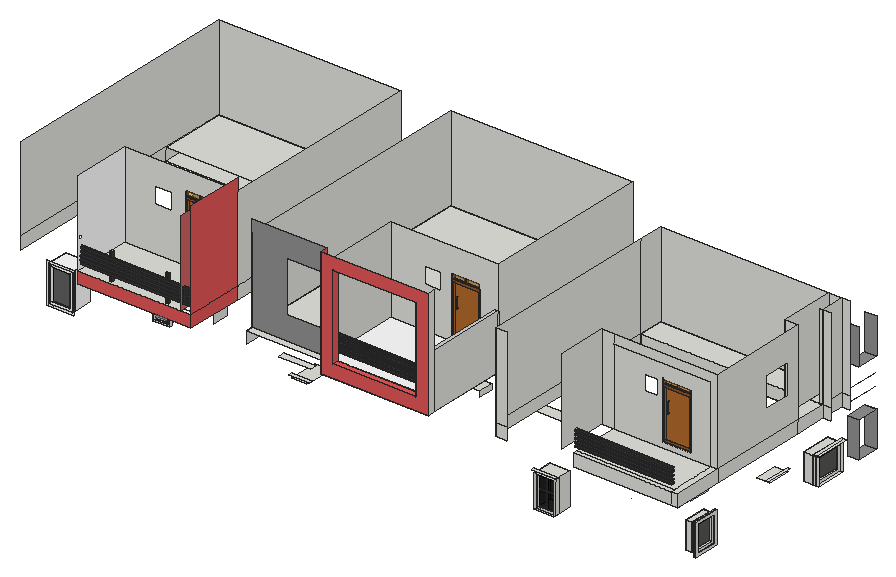
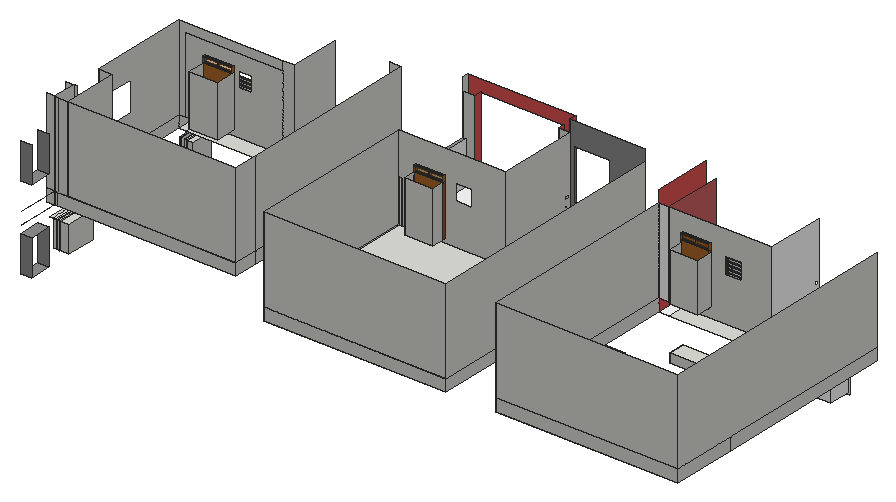
# SketchUp Ruby script. Lengths in inches.
U = 1.inch
M = Sketchup.active_model
def pt(a) = Geom::Point3d.new(a.map { |v| v * U })
def face(e, loops, mat)
  f = e.add_face(loops[0].map { |a| pt(a) })
  loops[1..].each { |l| e.add_face(l.map { |a| pt(a) }).erase! }
  f.material = f.back_material = mat if mat
  f
end
# faces: each face lists its corners as indices into pts; further lists are holes
def faces(e, pts, list, mat = nil) = list.each { |f| face(e, (f[0].is_a?(Array) ? f : [f]).map { |l| l.map { |i| pts[i] } }, mat) }
# xy, xz, yz: faces in a plane at the given z, y or x. An outline is a flat list of corners, or four numbers for a rectangle; further outlines are holes
def ring(l) = l.size == 4 ? [[l[0], l[1]], [l[2], l[1]], [l[2], l[3]], [l[0], l[3]]] : l.each_slice(2).to_a
def flat(e, list, mat, &to3) = list.each { |f| face(e, (f[0].is_a?(Array) ? f : [f]).map { |l| ring(l).map { |u, v| to3.(u, v) } }, mat) }
def xy(e, z, list, mat = nil) = flat(e, list, mat) { |x, y| [x, y, z] }
def xz(e, y, list, mat = nil) = flat(e, list, mat) { |x, z| [x, y, z] }
def yz(e, x, list, mat = nil) = flat(e, list, mat) { |y, z| [x, y, z] }
def lines(e, pts, list) = list.each { |a, b| e.add_line(pt(pts[a]), pt(pts[b])) }
# prism: a flat outline (further loops are holes) pulled along v
def prism(e, loops, v, mat = nil)
  f = face(e, loops, mat); d = Geom::Vector3d.new(v.map { |x| x * U })
  f.pushpull(f.normal.samedirection?(d) ? d.length : -d.length)
end
def box(e, o, s, mat = nil) = prism(e, [[o, [o[0] + s[0], o[1], o[2]], [o[0] + s[0], o[1] + s[1], o[2]], [o[0], o[1] + s[1], o[2]]]], [0, 0, s[2]], mat)
def at(x, y, z, deg = 0) = Geom::Transformation.translation(pt([x, y, z])) * Geom::Transformation.rotation(ORIGIN, Z_AXIS, deg.degrees)
def axes(o, x, y, z) = Geom::Transformation.new([*x, 0, *y, 0, *z, 0, *pt(o).to_a, 1])
def part(name) = M.definitions.add(name)
# library, detail: a bought-in or finely detailed component or shape, given as its bounding box
def library(name, o, s) = part(name).tap { |d| box(d.entities, o, s) }
def detail(e, o, s) = box(e.add_group.entities, o, s)
def put(e, d, t, mat = nil) = e.add_instance(d, t).tap { |i| i.material = mat if mat }
def group(e, t, mat = nil) = e.add_group.tap { |g| g.transformation = t; g.material = mat if mat }.entities
root = M.entities
M.materials.add("Generic").color = [145, 145, 145]
M.materials.add("Generic\#1").color = [206, 99, 99]
M.materials.add("Generic\#2").color = [229, 87, 87]
M.materials.add("[Color M00]").color = [255, 255, 255]
M.materials.add("[Color M07]").color = [58, 58, 58]
M.materials.add("[Color M08]").color = [45, 45, 45]
M.materials.add("[Translucent Glass Dark Green]").color = [168, 100, 12]
M.materials["[Translucent Glass Dark Green]"].alpha = 0.5
M.materials.add("[Translucent Glass Gray]").color = [0, 0, 0]
M.materials["[Translucent Glass Gray]"].alpha = 0.62
M.materials.add("[Translucent Glass Gray]1").color = [128, 128, 128]
M.materials["[Translucent Glass Gray]1"].alpha = 0.5
M.materials.add("[Wood Bamboo]").color = [177, 105, 43]
M.materials.add("[Wood Cherry Original]").color = [152, 86, 42]
c1 = part("Group\#1")
xy(c1.entities,0,[[0,0,39.9375,6]])
xy(c1.entities,3.79,[[3.79,0,36.15,3]])
xy(c1.entities,60.83,[[3.79,0,36.15,3]])
xy(c1.entities,64.62,[[0,0,39.9375,6]])
xz(c1.entities,0,[[[0,0,39.9375,64.62],[3.79,3.79,36.15,60.83]]])
xz(c1.entities,3,[[18.07,3.79,20.49,3.79,20.49,32.1,36.15,32.1,36.15,34.21,20.49,34.21,20.49,60.83,18.07,60.83,18.07,34.21,3.79,34.21,3.79,32.1,18.07,32.1]],"[Color M08]")
xz(c1.entities,3,[[3.79,3.79,18.07,32.1],[20.49,3.79,36.15,32.1],[3.79,34.21,18.07,60.83],[20.49,34.21,36.15,60.83]],"[Translucent Glass Gray]")
xz(c1.entities,6,[[0,0,39.9375,64.62]],"[Translucent Glass Gray]")
yz(c1.entities,0,[[0,0,6,64.62]])
yz(c1.entities,3.79,[[0,3.79,3,60.83]])
yz(c1.entities,36.15,[[0,3.79,3,60.83]])
yz(c1.entities,39.9375,[[0,0,6,64.62]])
c2 = part("Group\#8")
xy(c2.entities,0,[[0,0,6,59.4375]])
xy(c2.entities,4.64,[[3,4.64,6,54.8]])
xy(c2.entities,46.99,[[3,4.64,6,54.8]])
xy(c2.entities,51.625,[[0,0,6,59.4375]])
xz(c2.entities,0,[[0,0,6,51.625]])
xz(c2.entities,4.64,[[3,4.64,6,46.99]])
xz(c2.entities,54.8,[[3,4.64,6,46.99]])
xz(c2.entities,59.4375,[[0,0,6,51.625]])
yz(c2.entities,0,[[0,0,59.4375,51.625]])
yz(c2.entities,3,[[4.64,4.64,54.8,46.99]],"[Translucent Glass Gray]")
yz(c2.entities,6,[[[0,0,59.4375,51.625],[4.64,4.64,54.8,46.99]]])
c3 = part("Group\#11")
xy(c3.entities,0,[[0,0,27.8125,3]])
xy(c3.entities,27.8125,[[0,0,27.8125,3]])
xz(c3.entities,0,[[0,0,27.8125,27.8125]],"[Translucent Glass Gray]1")
xz(c3.entities,3,[[0,0,27.8125,27.8125]],"[Translucent Glass Gray]1")
yz(c3.entities,0,[[0,0,3,27.8125]])
yz(c3.entities,27.8125,[[0,0,3,27.8125]])
c4 = part("Group\#7")
xy(c4.entities,0,[[0,0,6,43.1875]])
xy(c4.entities,3.45,[[3,3.45,6,39.74]])
xy(c4.entities,49.61,[[3,3.45,6,39.74]])
xy(c4.entities,53.0625,[[0,0,6,43.1875]])
xz(c4.entities,0,[[0,0,6,53.0625]])
xz(c4.entities,3.45,[[3,3.45,6,49.61]])
xz(c4.entities,39.74,[[3,3.45,6,49.61]])
xz(c4.entities,43.1875,[[0,0,6,53.0625]])
yz(c4.entities,0,[[0,0,43.1875,53.0625]])
yz(c4.entities,3,[[3.45,3.45,39.74,49.61]],"[Translucent Glass Gray]")
yz(c4.entities,6,[[[0,0,43.1875,53.0625],[3.45,3.45,39.74,49.61]]])
c5 = part("Group\#5")
xy(c5.entities,0,[[0,0,46.6875,6]],"[Color M00]")
xy(c5.entities,4.48,[[4.48,0,42.2,3]],"[Color M00]")
xy(c5.entities,67.45,[[4.48,0,42.2,3]],"[Color M00]")
xy(c5.entities,71.9375,[[0,0,46.6875,6]],"[Color M00]")
xz(c5.entities,0,[[[0,0,46.6875,71.9375],[4.48,4.48,42.2,67.45]]],"[Color M00]")
xz(c5.entities,3,[[4.48,4.48,42.2,67.45]],"[Translucent Glass Gray]")
xz(c5.entities,6,[[0,0,46.6875,71.9375]],"[Color M00]")
yz(c5.entities,0,[[0,0,6,71.9375]],"[Color M00]")
yz(c5.entities,4.48,[[0,4.48,3,67.45]],"[Color M00]")
yz(c5.entities,42.2,[[0,4.48,3,67.45]],"[Color M00]")
yz(c5.entities,46.6875,[[0,0,6,71.9375]],"[Color M00]")
c6 = part("Group\#12")
xy(c6.entities,0,[[0,0,20.25,3]])
xy(c6.entities,24.8125,[[0,0,20.25,3]])
xz(c6.entities,0,[[0,0,20.25,24.8125]],"[Translucent Glass Gray]1")
xz(c6.entities,3,[[0,0,20.25,24.8125]],"[Translucent Glass Gray]1")
yz(c6.entities,0,[[0,0,3,24.8125]])
yz(c6.entities,20.25,[[0,0,3,24.8125]])
c7 = part("Group\#10")
xy(c7.entities,0,[[0,1.08,55.8125,6.01]],"[Wood Cherry Original]")
xy(c7.entities,3.96,[[3.96,1.08,51.86,3.01]],"[Wood Bamboo]")
xy(c7.entities,51.66,[[8.63,0,9.88,3.01]],"[Color M08]")
xy(c7.entities,52.54,[[8.63,0.6875,9.88,3.01]],"[Color M08]")
xy(c7.entities,71.82,[[8.63,0.6875,9.88,3.01]],"[Color M08]")
xy(c7.entities,72.69,[[8.63,0,9.88,3.01]],"[Color M08]")
xy(c7.entities,97.36,[[3.96,1.08,51.86,3.01]],"[Wood Bamboo]")
xy(c7.entities,101.3125,[[0,1.08,55.8125,6.01]],"[Wood Bamboo]")
xy(c7.entities,102.55,[[1.23,1.08,27.29,3.01],[27.29,1.08,28.52,1.95],[28.52,1.08,54.58,3.01]],"[Wood Bamboo]")
xy(c7.entities,112.31,[[1.23,1.08,1.23,3.01,27.29,3.01,27.29,1.95,28.52,1.95,28.52,3.01,54.58,3.01,54.58,1.08]],"[Wood Bamboo]")
xy(c7.entities,113.54,[[0,1.08,55.8125,6.01]],"[Wood Bamboo]")
xz(c7.entities,0,[[8.63,51.66,9.88,72.69]],"[Color M08]")
xz(c7.entities,0.6875,[[8.63,52.54,9.88,71.82]])
xz(c7.entities,1.08,[[0,101.3125,55.8125,102.55],[0,102.55,1.23,102.55,1.23,112.31,54.58,112.31,54.58,102.55,55.8125,102.55,55.8125,113.54,0,113.54]],"[Wood Bamboo]")
xz(c7.entities,1.08,[[[0,0,55.8125,101.3125],[3.96,3.96,51.86,97.36]]],"[Wood Cherry Original]")
xz(c7.entities,1.95,[[27.29,102.55,28.52,112.31]],"[Wood Bamboo]")
xz(c7.entities,3.01,[[8.63,71.82,9.88,72.69]])
xz(c7.entities,3.01,[[1.23,102.55,27.29,112.31],[28.52,102.55,54.58,112.31]],"[Translucent Glass Dark Green]")
xz(c7.entities,3.01,[[[3.96,3.96,51.86,97.36],[8.63,71.82,9.88,72.69],[8.63,51.66,9.88,52.54]]],"[Wood Bamboo]")
xz(c7.entities,6.01,[[0,0,55.8125,101.3125],[0,112.31,55.8125,113.54]],"[Wood Bamboo]")
yz(c7.entities,0,[[1.08,101.3125,6.01,113.54]],"[Wood Bamboo]")
yz(c7.entities,0,[[1.08,0,6.01,101.3125]],"[Wood Cherry Original]")
yz(c7.entities,1.23,[[1.08,102.55,3.01,112.31]],"[Wood Bamboo]")
yz(c7.entities,3.96,[[1.08,3.96,3.01,97.36]],"[Wood Bamboo]")
yz(c7.entities,8.63,[[0,51.66,0,72.69,3.01,72.69,3.01,71.82,0.6875,71.82,0.6875,52.54,3.01,52.54,3.01,51.66]],"[Color M08]")
yz(c7.entities,9.88,[[0,51.66,3.01,51.66,3.01,52.54,0.6875,52.54,0.6875,71.82,3.01,71.82,3.01,72.69,0,72.69]],"[Color M08]")
yz(c7.entities,27.29,[[1.95,102.55,3.01,112.31]],"[Wood Bamboo]")
yz(c7.entities,28.52,[[1.95,102.55,3.01,112.31]],"[Wood Bamboo]")
yz(c7.entities,51.86,[[1.08,3.96,3.01,97.36]],"[Wood Bamboo]")
yz(c7.entities,54.58,[[1.08,102.55,3.01,112.31]],"[Wood Bamboo]")
yz(c7.entities,55.8125,[[1.08,101.3125,6.01,113.54]],"[Wood Bamboo]")
yz(c7.entities,55.8125,[[1.08,0,6.01,101.3125]],"[Wood Cherry Original]")
p = [[1.23,3.01,112.31],[1.23,6.01,112.31],[9.24,3.01,71.99],[9.24,0.51,71.99],[9.24,0.51,52.37],[9.24,3.01,52.37]]
lines(c7.entities,p,[[0,1],[2,3],[3,4],[4,5]])
xy(root,644.75,[[1429.21,528.77,1451.02,572.96]],"Generic")
xy(root,645.13,[[1156.27,93.8125,1196.2,99.8125],[1156.27,99.8125,1196.2,134.3125]])
xy(root,647.24,[[1427.83,421.57,1452.58,481],[1452.58,421.57,1457.58,481]])
xy(root,650.36,[[1448.83,123.62,1452.83,175.61]])
xy(root,651.38,[[331.98,182.0625,365.3125,187.125]])
xy(root,654.13,[[334.74,182.0625,362.55,187.125],[334.74,187.125,362.55,221.125]])
xy(root,654.76,[[1430.27,128.02,1448.83,171.21],[1448.83,128.02,1452.83,171.21]])
xy(root,668.73,[[192.03,99.8125,238.71,141.8125]],"[Color M00]")
xy(root,670.4,[[808.05,253.75,841.375,258.8125]])
xy(root,673.16,[[810.81,253.75,838.62,258.8125],[810.81,258.8125,838.62,292.8125]])
xy(root,676.47,[[1292.01,194.1875,1317.77,199.25]])
xy(root,679.23,[[1294.76,194.1875,1315.01,199.25],[1294.76,199.25,1315.01,212.4375]])
xy(root,681.95,[[334.74,182.0625,362.55,187.125],[334.74,187.125,362.55,221.125]])
xy(root,684.7,[[331.98,182.0625,365.3125,187.125]])
xy(root,689.99,[[954.11,276.94,1080.05,298.38]])
xy(root,690.67,[[1414.21,322.92,1435.83,367.42],[1435.83,322.92,1439.83,367.42]])
xy(root,695.08,[[1435.83,318.51,1439.83,371.82]])
xy(root,698.86,[[1427.83,421.57,1452.58,481],[1452.58,421.57,1457.58,481]])
xy(root,699.22,[[862.05,258.8125,917.86,288.3125]])
xy(root,700.97,[[810.81,253.75,838.62,258.8125],[810.81,258.8125,838.62,292.8125]])
xy(root,702.28,[[392.26,187.125,448.07,220.9375]])
xy(root,703.27,[[1452.58,417.16,1457.58,485.41],[1457.58,417.16,1462.21,485.41]])
xy(root,703.73,[[808.05,253.75,841.375,258.8125]])
xy(root,704.04,[[1294.76,194.1875,1315.01,199.25],[1294.76,199.25,1315.01,212.4375]])
xy(root,706.34,[[1327.46,199.25,1383.27,240]])
xy(root,706.8,[[1292.01,194.1875,1317.77,199.25]])
xy(root,707.1875,[[495.5,271.33,593.5,290.83]])
xy(root,707.83,[[1430.27,128.02,1448.83,171.21],[1448.83,128.02,1452.83,171.21]])
xy(root,709.29,[[676.72,93.8125,707.97,99.8125],[676.72,99.8125,707.97,152.375]])
xy(root,709.75,[[1156.27,93.8125,1196.2,99.8125],[1156.27,99.8125,1196.2,134.3125]])
xy(root,712.23,[[1448.83,123.62,1452.83,175.61]])
xy(root,713.66,[[672.35,93.8125,712.33,99.8125]])
xy(root,714.12,[[1151.9,93.8125,1200.57,99.8125]])
xy(root,716.24,[[1429.21,528.77,1451.02,572.96]],"Generic")
xy(root,740.67,[[192.03,99.8125,238.71,141.8125]],"[Color M00]")
xy(root,744,[[272.78,71.5,475.8125,187.125],[657.35,86,720.59,99.8125],[741.96,86,954.11,99.8125],[741.96,99.8125,954.11,258.8125],[1230.96,99.8125,1423.39,199.25],
  [1423.39,99.8125,1435.83,199.25],[1427.83,398.12,1435.83,459.8125],[135.5,459.8125,495.5,590.625],[594.11,459.8125,954.11,590.625],[1075.83,459.8125,1427.83,507.75],
  [1427.83,459.8125,1435.83,507.75]])
xy(root,744,[[475.8125,71.5,495.5,187.125]],"[Color M00]")
xy(root,768,[[[272.78,71.5,475.8125,187.125],[333.5,76.97,335.06,81.1],[330.75,76.97,332.31,81.1],[445.18,76.97,446.75,79.72],[442.43,76.97,444,79.72]],[330.75,76.97,332.31,81.1],[333.5,76.97,335.06,81.1],[442.43,76.97,444,79.72],[445.18,76.97,446.75,79.72],
  [594.11,86,741.96,99.8125],[594.11,99.8125,594.11,459.8125,954.11,459.8125,954.11,258.8125,741.96,258.8125,741.96,99.8125],[1230.96,99.8125,1423.39,108.0625],[1423.39,99.8125,1435.83,199.25],[1230.96,108.0625,1423.39,199.25],
  [1409.33,398.12,1435.83,459.8125],[135.5,459.8125,495.5,590.625],[594.11,459.8125,954.11,590.625],[1075.83,459.8125,1409.33,507.75],[1409.33,459.8125,1435.83,507.75]])
xy(root,768,[[764.52,86,929.22,99.8125]],"Generic\#2")
xy(root,768,[[475.8125,71.5,495.5,79.5],[475.8125,79.5,495.5,187.125],[741.96,99.8125,947.55,258.8125]],"[Color M00]")
xy(root,776.27,[[862.0625,258.8125,917.875,288.3125]])
xy(root,778.5,[[1230.96,101.06,1423.39,106.62]],"[Color M07]")
xy(root,778.62,[[272.78,74.79,492.5625,80.4375]],"[Color M07]")
xy(root,778.74,[[741.96,106.52,947.55,111.34]],"[Color M07]")
xy(root,779.43,[[1327.46,199.25,1383.27,240]])
xy(root,780.62,[[741.96,106.52,947.55,111.34]],"[Color M07]")
xy(root,781.25,[[1230.96,101.06,1423.39,106.62]],"[Color M07]")
xy(root,782,[[272.78,74.79,492.5625,80.4375]],"[Color M07]")
xy(root,785.06,[[272.78,74.79,492.5625,80.4375]],"[Color M07]")
xy(root,785.4375,[[1230.96,101.06,1423.39,106.62]],"[Color M07]")
xy(root,785.81,[[741.96,106.52,947.55,111.34]],"[Color M07]")
xy(root,787.68,[[741.96,106.52,947.55,111.34]],"[Color M07]")
xy(root,788.1875,[[1230.96,101.06,1423.39,106.62]],"[Color M07]")
xy(root,788.43,[[272.78,74.79,492.5625,80.4375]],"[Color M07]")
xy(root,788.51,[[392.26,187.125,448.07,220.9375]])
xy(root,792.37,[[272.78,74.79,492.5625,80.4375]],"[Color M07]")
xy(root,792.4375,[[1230.96,101.06,1423.39,106.62]],"[Color M07]")
xy(root,793.24,[[741.96,106.52,947.55,111.34]],"[Color M07]")
xy(root,795.12,[[741.96,106.52,947.55,111.34]],"[Color M07]")
xy(root,795.1875,[[1230.96,101.06,1423.39,106.62]],"[Color M07]")
xy(root,795.75,[[272.78,74.79,492.5625,80.4375]],"[Color M07]")
xy(root,799.25,[[272.78,74.79,492.5625,80.4375]],"[Color M07]")
xy(root,799.6875,[[1230.96,101.06,1423.39,106.62]],"[Color M07]")
xy(root,799.99,[[741.96,106.52,947.55,111.34]],"[Color M07]")
xy(root,801.87,[[741.96,106.52,947.55,111.34]],"[Color M07]")
xy(root,802.4375,[[1230.96,101.06,1423.39,106.62]],"[Color M07]")
xy(root,802.62,[[272.78,74.79,492.5625,80.4375]],"[Color M07]")
xy(root,806.06,[[272.78,74.79,492.5625,80.4375]],"[Color M07]")
xy(root,806.5625,[[1230.96,101.06,1423.39,106.62]],"[Color M07]")
xy(root,807.31,[[741.96,106.52,947.55,111.34]],"[Color M07]")
xy(root,809.18,[[741.96,106.52,947.55,111.34]],"[Color M07]")
xy(root,809.3125,[[1230.96,101.06,1423.39,106.62]],"[Color M07]")
xy(root,809.43,[[272.78,74.79,492.5625,80.4375]],"[Color M07]")
xy(root,809.68,[[1429.21,528.77,1451.02,572.96]],"Generic")
xz(root,71.5,[[272.78,744,495.5,768]],"Generic\#2")
xz(root,74.79,[[272.78,778.62,492.5625,782],[272.78,785.06,492.5625,788.43],[272.78,792.37,492.5625,795.75],[272.78,799.25,492.5625,802.62],[272.78,806.06,492.5625,809.43]],"[Color M07]")
xz(root,76.97,[[330.75,768,332.31,821.06],[333.5,768,335.06,821.06],[442.43,768,444,821.06],[445.18,768,446.75,821.06]],"[Color M07]")
xz(root,79.72,[[442.43,768,444,821.06],[445.18,768,446.75,821.06]])
xz(root,80.4375,[[272.78,778.62,492.5625,782],[272.78,785.06,492.5625,788.43],[272.78,792.37,492.5625,795.75],[272.78,799.25,492.5625,802.62],[272.78,806.06,492.5625,809.43]])
xz(root,81.1,[[330.75,768,332.31,821.06],[333.5,768,335.06,821.06]])
xz(root,86,[[[741.96,744,954.11,960],[764.52,768,929.22,936]]],"Generic\#2")
xz(root,99.8125,[[741.96,744,741.96,768,947.55,768,947.55,852.8125,954.11,852.8125,954.11,744],[1075.83,744,1098.52,768],[1230.96,744,1423.39,768],[1423.39,744,1435.83,768],[741.96,768,764.52,936],
  [929.22,768,929.22,936,954.11,936,954.11,852.8125,947.55,852.8125,947.55,768],[1075.83,768,1098.52,936]])
xz(root,99.8125,[[[594.11,768,741.96,960],[663.18,813.78,734.35,915.58]]],"Generic")
xz(root,99.8125,[[[188.42,665.13,242.3125,744.27],[192.03,668.73,238.71,740.67]]],"[Color M00]")
xz(root,101.06,[[1230.96,778.5,1423.39,781.25],[1230.96,785.4375,1423.39,788.1875],[1230.96,792.4375,1423.39,795.1875],[1230.96,799.6875,1423.39,802.4375],[1230.96,806.5625,1423.39,809.3125]],"[Color M07]")
xz(root,106.52,[[741.96,778.74,947.55,780.62],[741.96,785.81,947.55,787.68],[741.96,793.24,947.55,795.12],[741.96,799.99,947.55,801.87],[741.96,807.31,947.55,809.18]],"[Color M07]")
xz(root,106.62,[[1230.96,778.5,1423.39,781.25],[1230.96,785.4375,1423.39,788.1875],[1230.96,792.4375,1423.39,795.1875],[1230.96,799.6875,1423.39,802.4375],[1230.96,806.5625,1423.39,809.3125]])
xz(root,111.34,[[741.96,778.74,947.55,780.62],[741.96,785.81,947.55,787.68],[741.96,793.24,947.55,795.12],[741.96,799.99,947.55,801.87],[741.96,807.31,947.55,809.18]])
xz(root,123.62,[[1448.83,650.36,1452.83,712.23]])
xz(root,128.02,[[1430.27,654.76,1448.83,707.83],[1448.83,654.76,1452.83,707.83]])
xz(root,134.3125,[[1156.27,645.13,1196.2,709.75]])
xz(root,141.8125,[[192.03,668.73,238.71,740.67]],"[Color M00]")
xz(root,171.21,[[1430.27,654.76,1448.83,707.83],[1448.83,654.76,1452.83,707.83]])
xz(root,175.61,[[1448.83,650.36,1452.83,712.23]])
xz(root,182.0625,[[[331.98,651.38,365.3125,684.7],[334.74,654.13,362.55,681.95]]])
xz(root,187.125,[[[331.98,651.38,365.3125,684.7],[334.74,654.13,362.55,681.95]],[[272.78,768,475.8125,936],[392.26,788.51,448.07,902.05],[331.98,855.44,365.3125,888.77]]])
xz(root,187.125,[[475.8125,768,495.5,936]],"[Color M00]")
xz(root,194.1875,[[[1292.01,676.47,1317.77,706.8],[1294.76,679.23,1315.01,704.04]]])
xz(root,199.25,[[[1292.01,676.47,1317.77,706.8],[1294.76,679.23,1315.01,704.04]],[1207.39,768,1230.96,936],[1423.39,768,1435.83,768,1435.83,936,1230.96,936,1230.96,917.875,1423.39,917.875],[[1230.96,768,1423.39,917.875],[1327.46,779.43,1383.27,890.49],[1292.01,856.66,1317.77,886.99]]])
xz(root,212.4375,[[1294.76,679.23,1315.01,704.04]])
xz(root,220.9375,[[392.26,683.84,448.07,702.28],[392.26,788.51,448.07,884.16]])
xz(root,221.125,[[334.74,654.13,362.55,681.95]])
xz(root,240,[[1327.46,693.68,1383.27,706.34],[1327.46,779.43,1383.27,880.74]])
xz(root,253.75,[[[808.05,670.4,841.375,703.73],[810.81,673.16,838.62,700.97]]])
xz(root,258.8125,[[[808.05,670.4,841.375,703.73],[810.81,673.16,838.62,700.97]],[[741.96,768,947.55,768,947.55,852.8125,954.11,852.8125,954.11,936,741.96,936],[862.0625,776.27,917.875,889.29],[808.05,849.34,841.375,882.67]]])
xz(root,258.8125,[[947.55,768,954.11,852.8125]],"[Color M00]")
xz(root,288.3125,[[862.05,688.43,917.86,699.22],[862.0625,776.27,917.875,877.58]])
xz(root,292.8125,[[810.81,673.16,838.62,700.97]])
xz(root,398.12,[[1409.33,768,1435.83,936]])
xz(root,421.57,[[1427.83,647.24,1452.58,698.86],[1452.58,647.24,1457.58,698.86]])
xz(root,459.8125,[[1075.83,744,1429.21,768],[1429.21,744,1433.58,768],[1433.58,744,1435.83,768],[1435.83,744,1451.02,768],[1429.21,768,1433.58,936],
  [1433.58,768,1435.83,936],[1435.83,768,1451.02,936]])
xz(root,481,[[1427.83,647.24,1452.58,698.86],[1452.58,647.24,1457.58,698.86]])
xz(root,507.75,[[1075.83,744,1429.21,768],[1429.21,744,1435.83,768],[1435.83,744,1451.02,768],[1075.83,768,1409.33,936],[1409.33,768,1429.21,936],
  [1429.21,768,1435.83,936],[1435.83,768,1451.02,936]])
xz(root,528.77,[[1429.21,644.75,1451.02,716.24],[1429.21,809.68,1451.02,881.18]],"Generic")
xz(root,572.96,[[1429.21,644.75,1451.02,716.24],[1429.21,809.68,1451.02,881.18]],"Generic")
xz(root,590.625,[[135.5,744,495.5,768],[594.11,744,954.11,768],[135.5,768,495.5,936],[594.11,768,954.11,936]])
yz(root,135.5,[[99.8125,744,459.8125,768],[459.8125,744,590.625,768],[99.8125,768,590.625,936]])
yz(root,192.03,[[99.8125,668.73,141.8125,740.67]],"[Color M00]")
yz(root,238.71,[[99.8125,668.73,141.8125,740.67]],"[Color M00]")
yz(root,272.78,[[74.79,778.62,80.4375,782],[74.79,785.06,80.4375,788.43],[74.79,792.37,80.4375,795.75],[74.79,799.25,80.4375,802.62],[74.79,806.06,80.4375,809.43]])
yz(root,272.78,[[[71.5,768,77.61,768,77.61,778.62,74.79,778.62,74.79,782,80.4375,782,80.4375,778.62,77.61,778.62,77.61,768,187.125,768,187.125,936,71.5,936],[72.41,821.06,80.4375,828.43],[74.79,785.06,80.4375,788.43],[74.79,792.37,80.4375,795.75],[74.79,799.25,80.4375,802.62],[74.79,806.06,80.4375,809.43]]],"[Color M00]")
yz(root,330.75,[[76.97,768,81.1,821.06]])
yz(root,331.98,[[182.0625,651.38,187.125,684.7]])
yz(root,332.31,[[76.97,768,81.1,821.06]],"[Color M07]")
yz(root,333.5,[[76.97,768,81.1,821.06]])
yz(root,334.74,[[182.0625,654.13,187.125,681.95],[187.125,654.13,221.125,681.95]])
yz(root,335.06,[[76.97,768,81.1,821.06]],"[Color M07]")
yz(root,362.55,[[182.0625,654.13,187.125,681.95],[187.125,654.13,221.125,681.95]])
yz(root,365.3125,[[182.0625,651.38,187.125,684.7]])
yz(root,392.26,[[187.125,683.84,220.9375,702.28],[187.125,788.51,220.9375,884.16]])
yz(root,442.43,[[76.97,768,79.72,821.06]],"[Color M07]")
yz(root,444,[[76.97,768,79.72,821.06]],"[Color M07]")
yz(root,445.18,[[76.97,768,79.72,821.06]],"[Color M07]")
yz(root,446.75,[[76.97,768,79.72,821.06]],"[Color M07]")
yz(root,448.07,[[187.125,683.84,220.9375,702.28],[187.125,788.51,220.9375,884.16]])
yz(root,475.8125,[[71.5,768,187.125,936]],"Generic\#1")
yz(root,492.5625,[[74.79,778.62,80.4375,782],[74.79,785.06,80.4375,788.43],[74.79,792.37,80.4375,795.75],[74.79,799.25,80.4375,802.62],[74.79,806.06,80.4375,809.43]])
yz(root,495.5,[[187.125,744,590.625,768],[187.125,768,590.625,936]])
yz(root,495.5,[[71.5,744,187.125,768],[71.5,768,187.125,960]],"Generic\#2")
yz(root,594.11,[[86,744,459.8125,768],[459.8125,744,590.625,768],[99.8125,768,590.625,936]])
yz(root,741.96,[[86,744,99.8125,768],[[99.8125,768,258.8125,936],[103.4,822.31,111.34,827.74],[106.52,778.74,111.34,780.62],[106.52,785.81,111.34,787.68],[106.52,793.24,111.34,795.12],[106.52,799.99,111.34,801.87],[106.52,807.31,111.34,809.18]],[106.52,778.74,111.34,780.62],[106.52,785.81,111.34,787.68],[106.52,793.24,111.34,795.12],
  [106.52,799.99,111.34,801.87],[106.52,807.31,111.34,809.18]])
yz(root,741.96,[[86,768,99.8125,960]],"Generic\#2")
yz(root,764.52,[[86,768,99.8125,936]],"Generic\#2")
yz(root,808.05,[[253.75,670.4,258.8125,703.73]])
yz(root,810.81,[[253.75,673.16,258.8125,700.97],[258.8125,673.16,292.8125,700.97]])
yz(root,838.62,[[253.75,673.16,258.8125,700.97],[258.8125,673.16,292.8125,700.97]])
yz(root,841.375,[[253.75,670.4,258.8125,703.73]])
yz(root,862.05,[[258.8125,688.43,288.3125,699.22]])
yz(root,862.0625,[[258.8125,776.27,288.3125,877.58]])
yz(root,917.86,[[258.8125,688.43,288.3125,699.22]])
yz(root,917.875,[[258.8125,776.27,288.3125,877.58]])
yz(root,929.22,[[86,768,99.8125,936]],"Generic\#2")
yz(root,947.55,[[[99.8125,768,258.8125,852.8125],[103.4,822.31,111.34,827.74],[106.52,807.31,111.34,809.18],[106.52,799.99,111.34,801.87],[106.52,793.24,111.34,795.12],[106.52,785.81,111.34,787.68],[106.52,778.74,111.34,780.62]]],"[Color M00]")
yz(root,954.11,[[86,744,99.8125,960],[99.8125,744,260.5,744,260.5,768,258.8125,768,258.8125,852.8125,99.8125,852.8125],[260.5,744,590.625,768],[258.8125,768,260.5,852.8125],[260.5,768,590.625,936]])
yz(root,1075.83,[[99.8125,744,459.8125,768],[459.8125,744,507.75,768],[99.8125,768,459.8125,936],[459.8125,768,507.75,936]])
yz(root,1156.27,[[93.8125,645.13,99.8125,709.75],[99.8125,645.13,134.3125,709.75]])
yz(root,1196.2,[[93.8125,645.13,99.8125,709.75],[99.8125,645.13,134.3125,709.75]])
yz(root,1207.39,[[99.8125,768,199.25,936]])
yz(root,1230.96,[[101.06,778.5,106.62,781.25],[101.06,785.4375,106.62,788.1875],[101.06,792.4375,106.62,795.1875],[101.06,799.6875,106.62,802.4375],[101.06,806.5625,106.62,809.3125]])
yz(root,1292.01,[[194.1875,676.47,199.25,706.8]])
yz(root,1294.76,[[194.1875,679.23,199.25,704.04],[199.25,679.23,212.4375,704.04]])
yz(root,1315.01,[[194.1875,679.23,199.25,704.04],[199.25,679.23,212.4375,704.04]])
yz(root,1317.77,[[194.1875,676.47,199.25,706.8]])
yz(root,1327.46,[[199.25,693.68,240,706.34],[199.25,779.43,240,880.74]])
yz(root,1383.27,[[199.25,693.68,240,706.34],[199.25,779.43,240,880.74]])
yz(root,1409.33,[[398.12,768,507.75,936]])
yz(root,1427.83,[[421.57,647.24,481,698.86]])
yz(root,1430.27,[[128.02,654.76,171.21,707.83]])
yz(root,1435.83,[[99.8125,744,199.25,768],[199.25,744,398.12,768],[398.12,744,459.8125,768],[459.8125,744,507.75,768],[[199.25,768,398.12,936],[318.51,823.02,371.82,881.83]],
  [459.8125,768,507.75,936]])
yz(root,1448.83,[[[123.62,650.36,175.61,712.23],[128.02,654.76,171.21,707.83]]])
yz(root,1452.83,[[[123.62,650.36,175.61,712.23],[128.02,654.76,171.21,707.83]]])
p = [[272.78,77.5,780],[475.8125,77.5,780],[272.78,77.5,787],[475.8125,77.5,787],[272.78,77.5,794],[475.8125,77.5,794],
  [272.78,77.5,801],[475.8125,77.5,801],[272.78,77.5,808],[475.8125,77.5,808],[332.78,77.61,778.62],[332.78,77.61,768],
  [1435.83,507.75,768],[1435.83,590.625,768],[741.96,108.79,780],[947.55,108.79,780],[741.96,108.79,787],[947.55,108.79,787],
  [741.96,108.79,794],[947.55,108.79,794],[741.96,108.79,801],[947.55,108.79,801],[741.96,108.79,808],[947.55,108.79,808],
  [1230.96,103.9375,780],[1423.39,103.9375,780],[1230.96,103.9375,787],[1423.39,103.9375,787],[1230.96,103.9375,794],[1423.39,103.9375,794],
  [1230.96,103.9375,801],[1423.39,103.9375,801],[1230.96,103.9375,808],[1423.39,103.9375,808],[1264.98,199.25,690.33],[1264.92,199.25,690.33],
  [1264.92,199.25,656.33],[1264.98,199.25,656.33],[1435.83,507.75,744],[1435.83,590.625,744]]
lines(root,p,[[0,1],[2,3],[4,5],[6,7],[8,9],[10,11],[12,13],[14,15],[16,17],[18,19],[20,21],[22,23],
  [24,25],[26,27],[28,29],[30,31],[32,33],[34,35],[36,37],[38,39]])
put(root,c1,at(1156.27,99.8125,645.13))
put(root,c2,at(1446.58,421.57,647.24))
put(root,c3,at(334.74,187.125,654.13))
put(root,c4,at(1442.83,128.02,654.76))
put(root,c5,at(192.03,99.8125,668.73))
put(root,c3,at(810.81,258.8125,673.16))
put(root,c6,at(1294.76,199.25,679.23))
put(root,c7,at(862.0625,258.8125,775.91))
put(root,c7,at(1327.46,199.25,779.43))
put(root,c7,at(392.26,187.125,788.51))
